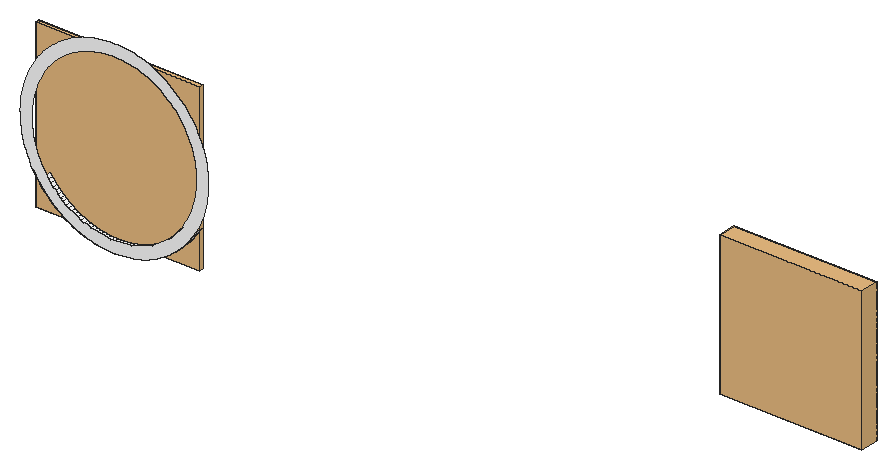
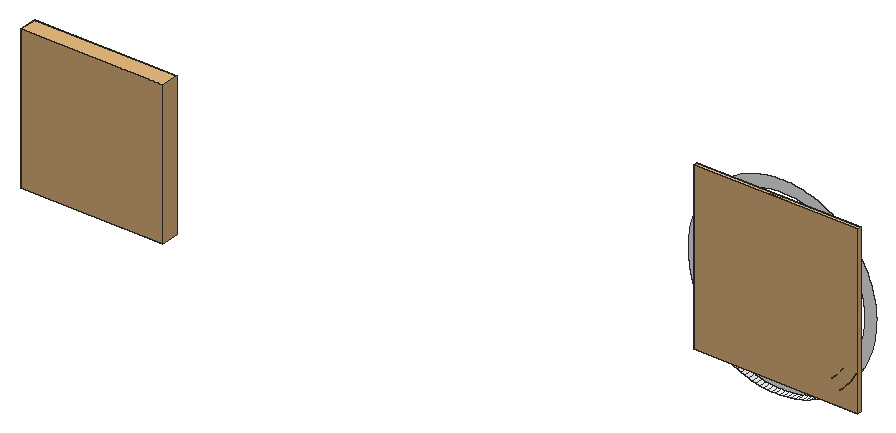
# SketchUp Ruby script. Lengths in inches.
U = 1.inch
M = Sketchup.active_model
def pt(a) = Geom::Point3d.new(a.map { |v| v * U })
def face(e, loops, mat)
  f = e.add_face(loops[0].map { |a| pt(a) })
  loops[1..].each { |l| e.add_face(l.map { |a| pt(a) }).erase! }
  f.material = f.back_material = mat if mat
  f
end
# faces: each face lists its corners as indices into pts; further lists are holes
def faces(e, pts, list, mat = nil) = list.each { |f| face(e, (f[0].is_a?(Array) ? f : [f]).map { |l| l.map { |i| pts[i] } }, mat) }
# xy, xz, yz: faces in a plane at the given z, y or x. An outline is a flat list of corners, or four numbers for a rectangle; further outlines are holes
def ring(l) = l.size == 4 ? [[l[0], l[1]], [l[2], l[1]], [l[2], l[3]], [l[0], l[3]]] : l.each_slice(2).to_a
def flat(e, list, mat, &to3) = list.each { |f| face(e, (f[0].is_a?(Array) ? f : [f]).map { |l| ring(l).map { |u, v| to3.(u, v) } }, mat) }
def xy(e, z, list, mat = nil) = flat(e, list, mat) { |x, y| [x, y, z] }
def xz(e, y, list, mat = nil) = flat(e, list, mat) { |x, z| [x, y, z] }
def yz(e, x, list, mat = nil) = flat(e, list, mat) { |y, z| [x, y, z] }
def lines(e, pts, list) = list.each { |a, b| e.add_line(pt(pts[a]), pt(pts[b])) }
# prism: a flat outline (further loops are holes) pulled along v
def prism(e, loops, v, mat = nil)
  f = face(e, loops, mat); d = Geom::Vector3d.new(v.map { |x| x * U })
  f.pushpull(f.normal.samedirection?(d) ? d.length : -d.length)
end
def box(e, o, s, mat = nil) = prism(e, [[o, [o[0] + s[0], o[1], o[2]], [o[0] + s[0], o[1] + s[1], o[2]], [o[0], o[1] + s[1], o[2]]]], [0, 0, s[2]], mat)
def at(x, y, z, deg = 0) = Geom::Transformation.translation(pt([x, y, z])) * Geom::Transformation.rotation(ORIGIN, Z_AXIS, deg.degrees)
def axes(o, x, y, z) = Geom::Transformation.new([*x, 0, *y, 0, *z, 0, *pt(o).to_a, 1])
def part(name) = M.definitions.add(name)
# library, detail: a bought-in or finely detailed component or shape, given as its bounding box
def library(name, o, s) = part(name).tap { |d| box(d.entities, o, s) }
def detail(e, o, s) = box(e.add_group.entities, o, s)
def put(e, d, t, mat = nil) = e.add_instance(d, t).tap { |i| i.material = mat if mat }
def group(e, t, mat = nil) = e.add_group.tap { |g| g.transformation = t; g.material = mat if mat }.entities
root = M.entities
M.materials.add("Leather White 002 15.0cm").color = [255, 255, 255]
M.materials.add("Wood 012 27.21cm").color = [255, 255, 255]
c1 = library("Window Crafter Sliding 2",[0,-0.55,0],[36,4.49,36])
c2 = library("Group622\#1",[-20.88,-20.88,0],[41.58,41.76,1])
xz(root,48.93,[[[33.9,178.41,34.89,178.43,35.89,178.5,36.875,178.61,37.86,178.76,38.84,178.95,39.8,179.18,40.76,179.45,41.7,179.77,42.63,180.12,43.55,180.51,44.45,180.9375,45.33,181.4,46.19,181.9,47.02,182.44,47.84,183.01,48.625,183.62,49.39,184.26,50.125,184.93,50.83,185.625,51.51,186.35,52.16,187.11,52.77,187.89,53.35,188.7,53.9,189.53,54.41,190.39,54.88,191.26,55.32,192.15,55.72,193.0625,56.08,193.99,56.4,194.93,56.69,195.89,56.93,196.85,57.13,197.82,57.29,198.81,57.41,199.79,57.49,200.79,57.52,201.78,57.52,202.77,57.47,203.77,57.38,204.76,57.25,205.75,57.08,206.73,56.87,207.7,56.62,208.66,56.33,209.61,56,210.55,55.625,211.47,55.22,212.38,54.77,213.27,54.28,214.14,53.77,214.98,53.21,215.81,52.62,216.61,52,217.39,51.35,218.14,50.66,218.86,49.95,219.55,49.2,220.21,48.43,220.84,47.64,221.44,46.82,222,45.98,222.53,45.11,223.03,44.23,223.48,43.33,223.9,42.41,224.28,41.47,224.625,40.53,224.93,39.57,225.1875,38.6,225.41,37.62,225.59,36.63,225.73,35.64,225.83,34.65,225.89,33.66,225.91,32.66,225.88,31.67,225.8125,30.68,225.7,29.7,225.55,28.72,225.36,27.75,225.13,26.8,224.86,25.85,224.54,24.92,224.19,24.01,223.8,23.11,223.375,22.23,222.91,21.37,222.41,20.53,221.87,19.72,221.3,18.93,220.69,18.17,220.05,17.43,219.38,16.72,218.68,16.05,217.96,15.4,217.2,14.79,216.42,14.21,215.61,13.66,214.78,13.15,213.92,12.67,213.05,12.24,212.16,11.84,211.25,11.48,210.32,11.15,209.38,10.87,208.42,10.63,207.46,10.43,206.49,10.27,205.5,10.15,204.52,10.07,203.52,10.03,202.53,10.04,201.54,10.08,200.54,10.17,199.55,10.3,198.57,10.47,197.59,10.68,196.61,10.9375,195.65,11.23,194.7,11.56,193.76,11.93,192.84,12.34,191.93,12.79,191.04,13.27,190.17,13.79,189.33,14.35,188.5,14.93,187.7,15.56,186.92,16.21,186.17,16.89,185.45,17.61,184.76,18.35,184.1,19.12,183.47,19.92,182.87,20.74,182.31,21.58,181.78,22.44,181.28,23.33,180.83,24.23,180.41,25.15,180.03,26.08,179.6875,27.03,179.38,27.99,179.12,28.96,178.9,29.9375,178.72,30.92,178.58,31.91,178.48,32.91,178.42],[33.89,181.27,33.01,181.29,32.14,181.34,31.27,181.43,30.4,181.55,29.54,181.71,28.6875,181.9,27.85,182.13,27.01,182.4,26.19,182.7,25.38,183.04,24.59,183.4,23.8125,183.81,23.05,184.24,22.3125,184.7,21.59,185.2,20.89,185.72,20.22,186.28,19.5625,186.86,18.93,187.47,18.33,188.1,17.76,188.76,17.21,189.45,16.69,190.15,16.21,190.875,15.75,191.62,15.32,192.39,14.93,193.17,14.57,193.96,14.24,194.78,13.95,195.6,13.7,196.4375,13.47,197.28,13.29,198.14,13.14,199,13.02,199.87,12.95,200.74,12.9,201.61,12.9,202.49,12.93,203.36,13,204.23,13.11,205.1,13.25,205.96,13.42,206.82,13.64,207.67,13.89,208.51,14.17,209.33,14.49,210.15,14.84,210.95,15.22,211.73,15.64,212.5,16.09,213.25,16.57,213.98,17.08,214.69,17.62,215.38,18.1875,216.05,18.78,216.6875,19.41,217.3,20.05,217.89,20.72,218.45,21.42,218.99,22.13,219.49,22.87,219.96,23.625,220.4,24.4,220.8125,25.1875,221.1875,25.99,221.53,26.81,221.84,27.64,222.11,28.48,222.35,29.33,222.56,30.19,222.73,31.05,222.86,31.92,222.95,32.8,223.01,33.67,223.04,34.55,223.02,35.42,222.97,36.29,222.88,37.15,222.76,38.01,222.6,38.87,222.41,39.71,222.18,40.54,221.91,41.36,221.61,42.17,221.27,42.97,220.91,43.74,220.5,44.5,220.07,45.24,219.61,45.96,219.11,46.66,218.59,47.34,218.03,47.99,217.45,48.62,216.84,49.22,216.21,49.8,215.55,50.35,214.87,50.86,214.16,51.35,213.43,51.81,212.6875,52.23,211.92,52.625,211.14,52.99,210.35,53.3125,209.53,53.6,208.71,53.86,207.875,54.08,207.03,54.27,206.17,54.42,205.3125,54.53,204.44,54.61,203.57,54.65,202.7,54.66,201.83,54.625,200.95,54.56,200.08,54.45,199.21,54.31,198.35,54.13,197.49,53.92,196.64,53.67,195.8,53.39,194.98,53.07,194.16,52.72,193.36,52.33,192.58,51.91,191.81,51.47,191.06,50.99,190.33,50.47,189.62,49.94,188.93,49.37,188.26,48.77,187.62,48.15,187.01,47.5,186.42,46.83,185.86,46.14,185.33,45.42,184.82,44.6875,184.35,43.93,183.91,43.16,183.5,42.37,183.125,41.5625,182.78,40.75,182.47,39.92,182.2,39.07,181.96,38.22,181.75,37.37,181.58,36.5,181.45,35.63,181.36,34.76,181.3]]],"Leather White 002 15.0cm")
xz(root,50.93,[[33.89,181.27,34.76,181.3,35.63,181.36,36.5,181.45,37.37,181.58,38.22,181.75,39.07,181.96,39.92,182.2,40.75,182.47,41.5625,182.78,42.37,183.125,43.16,183.5,43.93,183.91,44.6875,184.35,45.42,184.82,46.14,185.33,46.83,185.86,47.5,186.42,48.15,187.01,48.77,187.62,49.37,188.26,49.94,188.93,50.47,189.62,50.99,190.33,51.47,191.06,51.91,191.81,52.33,192.58,52.72,193.36,53.07,194.16,53.39,194.98,53.67,195.8,53.92,196.64,54.13,197.49,54.31,198.35,54.45,199.21,54.56,200.08,54.625,200.95,54.66,201.83,54.65,202.7,54.61,203.57,54.53,204.44,54.42,205.3125,54.27,206.17,54.08,207.03,53.86,207.875,53.6,208.71,53.3125,209.53,52.99,210.35,52.625,211.14,52.23,211.92,51.81,212.6875,51.35,213.43,50.86,214.16,50.35,214.87,49.8,215.55,49.22,216.21,48.62,216.84,47.99,217.45,47.34,218.03,46.66,218.59,45.96,219.11,45.24,219.61,44.5,220.07,43.74,220.5,42.97,220.91,42.17,221.27,41.36,221.61,40.54,221.91,39.71,222.18,38.87,222.41,38.01,222.6,37.15,222.76,36.29,222.88,35.42,222.97,34.55,223.02,33.67,223.04,32.8,223.01,31.92,222.95,31.05,222.86,30.19,222.73,29.33,222.56,28.48,222.35,27.64,222.11,26.81,221.84,25.99,221.53,25.1875,221.1875,24.4,220.8125,23.625,220.4,22.87,219.96,22.13,219.49,21.42,218.99,20.72,218.45,20.05,217.89,19.41,217.3,18.78,216.6875,18.1875,216.05,17.62,215.38,17.08,214.69,16.57,213.98,16.09,213.25,15.64,212.5,15.22,211.73,14.84,210.95,14.49,210.15,14.17,209.33,13.89,208.51,13.64,207.67,13.42,206.82,13.25,205.96,13.11,205.1,13,204.23,12.93,203.36,12.9,202.49,12.9,201.61,12.95,200.74,13.02,199.87,13.14,199,13.29,198.14,13.47,197.28,13.7,196.4375,13.95,195.6,14.24,194.78,14.57,193.96,14.93,193.17,15.32,192.39,15.75,191.62,16.21,190.875,16.69,190.15,17.21,189.45,17.76,188.76,18.33,188.1,18.93,187.47,19.5625,186.86,20.22,186.28,20.89,185.72,21.59,185.2,22.3125,184.7,23.05,184.24,23.8125,183.81,24.59,183.4,25.38,183.04,26.19,182.7,27.01,182.4,27.85,182.13,28.6875,181.9,29.54,181.71,30.4,181.55,31.27,181.43,32.14,181.34,33.01,181.29]])
p = [[31.91,50.93,178.48],[32.91,50.93,178.42],[32.91,48.93,178.42],[31.91,48.93,178.48],[33.9,50.93,178.41],[33.9,48.93,178.41],
  [34.89,50.93,178.43],[34.89,48.93,178.43],[35.89,50.93,178.5],[35.89,48.93,178.5],[30.92,50.93,178.58],[30.92,48.93,178.58],
  [36.875,50.93,178.61],[36.875,48.93,178.61],[29.9375,50.93,178.72],[29.9375,48.93,178.72],[37.86,50.93,178.76],[37.86,48.93,178.76],
  [28.96,50.93,178.9],[28.96,48.93,178.9],[38.84,50.93,178.95],[38.84,48.93,178.95],[27.99,50.93,179.12],[27.99,48.93,179.12],
  [39.8,50.93,179.18],[39.8,48.93,179.18],[27.03,50.93,179.38],[27.03,48.93,179.38],[40.76,50.93,179.45],[40.76,48.93,179.45],
  [26.08,50.93,179.6875],[26.08,48.93,179.6875],[41.7,50.93,179.77],[41.7,48.93,179.77],[25.15,50.93,180.03],[25.15,48.93,180.03],
  [42.63,50.93,180.12],[42.63,48.93,180.12],[24.23,50.93,180.41],[24.23,48.93,180.41],[43.55,50.93,180.51],[43.55,48.93,180.51],
  [23.33,50.93,180.83],[23.33,48.93,180.83],[44.45,50.93,180.9375],[44.45,48.93,180.9375],[22.44,50.93,181.28],[22.44,48.93,181.28],
  [45.33,50.93,181.4],[45.33,48.93,181.4],[21.58,50.93,181.78],[21.58,48.93,181.78],[32.14,50.93,181.34],[31.27,50.93,181.43],
  [31.27,48.93,181.43],[32.14,48.93,181.34],[33.01,50.93,181.29],[33.01,48.93,181.29],[33.89,50.93,181.27],[33.89,48.93,181.27],
  [34.76,50.93,181.3],[34.76,48.93,181.3],[35.63,50.93,181.36],[35.63,48.93,181.36],[30.4,50.93,181.55],[30.4,48.93,181.55],
  [36.5,50.93,181.45],[36.5,48.93,181.45],[46.19,50.93,181.9],[46.19,48.93,181.9],[29.54,50.93,181.71],[29.54,48.93,181.71],
  [37.37,50.93,181.58],[37.37,48.93,181.58],[38.22,50.93,181.75],[38.22,48.93,181.75],[28.6875,50.93,181.9],[28.6875,48.93,181.9],
  [20.74,50.93,182.31],[20.74,48.93,182.31],[39.07,50.93,181.96],[39.07,48.93,181.96],[27.85,50.93,182.13],[27.85,48.93,182.13],
  [47.02,50.93,182.44],[47.02,48.93,182.44],[39.92,50.93,182.2],[39.92,48.93,182.2],[27.01,50.93,182.4],[27.01,48.93,182.4],
  [40.75,50.93,182.47],[40.75,48.93,182.47],[19.92,50.93,182.87],[19.92,48.93,182.87],[26.19,50.93,182.7],[26.19,48.93,182.7],
  [47.84,50.93,183.01],[47.84,48.93,183.01],[41.5625,50.93,182.78],[41.5625,48.93,182.78],[25.38,50.93,183.04],[25.38,48.93,183.04],
  [42.37,50.93,183.125],[42.37,48.93,183.125],[19.12,50.93,183.47],[19.12,48.93,183.47],[24.59,50.93,183.4],[24.59,48.93,183.4],
  [48.625,50.93,183.62],[48.625,48.93,183.62],[43.16,50.93,183.5],[43.16,48.93,183.5],[23.8125,50.93,183.81],[23.8125,48.93,183.81],
  [18.35,50.93,184.1],[18.35,48.93,184.1],[43.93,50.93,183.91],[43.93,48.93,183.91],[49.39,50.93,184.26],[49.39,48.93,184.26],
  [23.05,50.93,184.24],[23.05,48.93,184.24],[44.6875,50.93,184.35],[44.6875,48.93,184.35],[17.61,50.93,184.76],[17.61,48.93,184.76],
  [22.3125,50.93,184.7],[22.3125,48.93,184.7],[50.125,50.93,184.93],[50.125,48.93,184.93],[45.42,50.93,184.82],[45.42,48.93,184.82],
  [21.59,50.93,185.2],[21.59,48.93,185.2],[16.89,50.93,185.45],[16.89,48.93,185.45],[46.14,50.93,185.33],[46.14,48.93,185.33],
  [50.83,50.93,185.625],[50.83,48.93,185.625],[20.89,50.93,185.72],[20.89,48.93,185.72],[46.83,50.93,185.86],[46.83,48.93,185.86],
  [16.21,50.93,186.17],[16.21,48.93,186.17],[51.51,50.93,186.35],[51.51,48.93,186.35],[20.22,50.93,186.28],[20.22,48.93,186.28],
  [47.5,50.93,186.42],[47.5,48.93,186.42],[15.56,50.93,186.92],[15.56,48.93,186.92],[19.5625,50.93,186.86],[19.5625,48.93,186.86],
  [48.15,50.93,187.01],[48.15,48.93,187.01],[52.16,50.93,187.11],[52.16,48.93,187.11],[14.93,50.93,187.7],[14.93,48.93,187.7],
  [18.93,50.93,187.47],[18.93,48.93,187.47],[48.77,50.93,187.62],[48.77,48.93,187.62],[52.77,50.93,187.89],[52.77,48.93,187.89],
  [18.33,50.93,188.1],[18.33,48.93,188.1],[49.37,50.93,188.26],[49.37,48.93,188.26],[14.35,50.93,188.5],[14.35,48.93,188.5],
  [53.35,50.93,188.7],[53.35,48.93,188.7],[17.76,50.93,188.76],[17.76,48.93,188.76],[49.94,50.93,188.93],[49.94,48.93,188.93],
  [13.79,50.93,189.33],[13.79,48.93,189.33],[53.9,50.93,189.53],[53.9,48.93,189.53],[17.21,50.93,189.45],[17.21,48.93,189.45],
  [50.47,50.93,189.62],[50.47,48.93,189.62],[13.27,50.93,190.17],[13.27,48.93,190.17],[16.69,50.93,190.15],[16.69,48.93,190.15],
  [54.41,50.93,190.39],[54.41,48.93,190.39],[50.99,50.93,190.33],[50.99,48.93,190.33]]
faces(root,p,[[0,1,2,3],[1,4,5,2],[4,6,7,5],[6,8,9,7],[10,0,3,11],[8,12,13,9],[14,10,11,15],[12,16,17,13],
  [18,14,15,19],[16,20,21,17],[22,18,19,23],[20,24,25,21],[26,22,23,27],[24,28,29,25],[30,26,27,31],[28,32,33,29],
  [34,30,31,35],[32,36,37,33],[38,34,35,39],[36,40,41,37],[42,38,39,43],[40,44,45,41],[46,42,43,47],[44,48,49,45],
  [50,46,47,51],[52,53,54,55],[56,52,55,57],[58,56,57,59],[60,58,59,61],[62,60,61,63],[53,64,65,54],[66,62,63,67],
  [48,68,69,49],[64,70,71,65],[72,66,67,73],[74,72,73,75],[70,76,77,71],[78,50,51,79],[80,74,75,81],[76,82,83,77],
  [68,84,85,69],[86,80,81,87],[82,88,89,83],[90,86,87,91],[92,78,79,93],[88,94,95,89],[84,96,97,85],[98,90,91,99],
  [94,100,101,95],[102,98,99,103],[104,92,93,105],[100,106,107,101],[96,108,109,97],[110,102,103,111],[106,112,113,107],[114,104,105,115],
  [116,110,111,117],[108,118,119,109],[112,120,121,113],[122,116,117,123],[124,114,115,125],[120,126,127,121],[118,128,129,119],[130,122,123,131],
  [126,132,133,127],[134,124,125,135],[136,130,131,137],[128,138,139,129],[132,140,141,133],[142,136,137,143],[144,134,135,145],[138,146,147,139],
  [140,148,149,141],[150,142,143,151],[152,144,145,153],[148,154,155,149],[156,150,151,157],[146,158,159,147],[160,152,153,161],[154,162,163,155],
  [164,156,157,165],[158,166,167,159],[162,168,169,163],[170,164,165,171],[172,160,161,173],[166,174,175,167],[168,176,177,169],[178,170,171,179],
  [180,172,173,181],[174,182,183,175],[176,184,185,177],[186,178,179,187],[188,180,181,189],[184,190,191,185],[182,192,193,183],[194,186,187,195]],"Leather White 002 15.0cm")
put(root,c1,at(164.22,77.74,180))
put(root,c2,axes([33.8,51.09,202.07],[1,0,0],[0,0,1],[0,-1,0]),"Wood 012 27.21cm")
